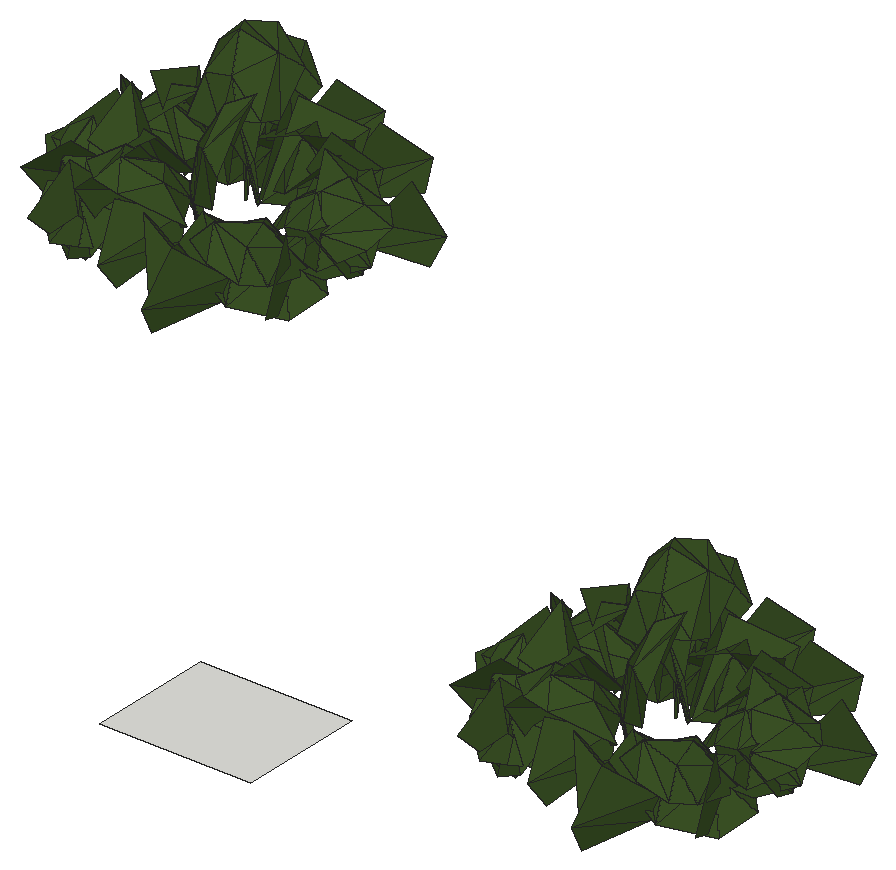
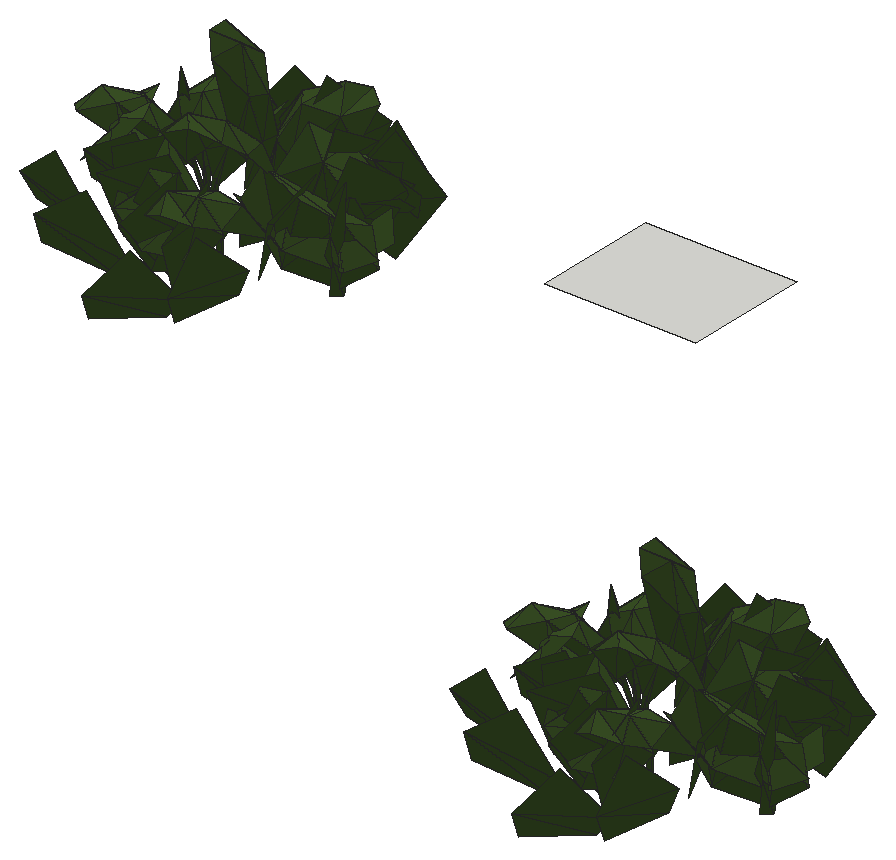
# SketchUp Ruby script. Lengths in inches.
U = 1.inch
M = Sketchup.active_model
def pt(a) = Geom::Point3d.new(a.map { |v| v * U })
def face(e, loops, mat)
  f = e.add_face(loops[0].map { |a| pt(a) })
  loops[1..].each { |l| e.add_face(l.map { |a| pt(a) }).erase! }
  f.material = f.back_material = mat if mat
  f
end
# faces: each face lists its corners as indices into pts; further lists are holes
def faces(e, pts, list, mat = nil) = list.each { |f| face(e, (f[0].is_a?(Array) ? f : [f]).map { |l| l.map { |i| pts[i] } }, mat) }
# xy, xz, yz: faces in a plane at the given z, y or x. An outline is a flat list of corners, or four numbers for a rectangle; further outlines are holes
def ring(l) = l.size == 4 ? [[l[0], l[1]], [l[2], l[1]], [l[2], l[3]], [l[0], l[3]]] : l.each_slice(2).to_a
def flat(e, list, mat, &to3) = list.each { |f| face(e, (f[0].is_a?(Array) ? f : [f]).map { |l| ring(l).map { |u, v| to3.(u, v) } }, mat) }
def xy(e, z, list, mat = nil) = flat(e, list, mat) { |x, y| [x, y, z] }
def xz(e, y, list, mat = nil) = flat(e, list, mat) { |x, z| [x, y, z] }
def yz(e, x, list, mat = nil) = flat(e, list, mat) { |y, z| [x, y, z] }
def lines(e, pts, list) = list.each { |a, b| e.add_line(pt(pts[a]), pt(pts[b])) }
# prism: a flat outline (further loops are holes) pulled along v
def prism(e, loops, v, mat = nil)
  f = face(e, loops, mat); d = Geom::Vector3d.new(v.map { |x| x * U })
  f.pushpull(f.normal.samedirection?(d) ? d.length : -d.length)
end
def box(e, o, s, mat = nil) = prism(e, [[o, [o[0] + s[0], o[1], o[2]], [o[0] + s[0], o[1] + s[1], o[2]], [o[0], o[1] + s[1], o[2]]]], [0, 0, s[2]], mat)
def at(x, y, z, deg = 0) = Geom::Transformation.translation(pt([x, y, z])) * Geom::Transformation.rotation(ORIGIN, Z_AXIS, deg.degrees)
def axes(o, x, y, z) = Geom::Transformation.new([*x, 0, *y, 0, *z, 0, *pt(o).to_a, 1])
def part(name) = M.definitions.add(name)
# library, detail: a bought-in or finely detailed component or shape, given as its bounding box
def library(name, o, s) = part(name).tap { |d| box(d.entities, o, s) }
def detail(e, o, s) = box(e.add_group.entities, o, s)
def put(e, d, t, mat = nil) = e.add_instance(d, t).tap { |i| i.material = mat if mat }
def group(e, t, mat = nil) = e.add_group.tap { |g| g.transformation = t; g.material = mat if mat }.entities
root = M.entities
M.materials.add("AM113_062_Tilia").color = [58, 81, 37]
xy(root,701.22,[[935.92,76.875,1160.625,265.5]])
p = [[1326.61,433.49,700.58],[1335.91,414.52,720.31],[1282.43,508.64,794.36],[1285.77,510.27,749.37],[165.99,1082.26,700.58],[175.28,1063.3,720.31],
  [121.81,1157.41,794.36],[125.14,1159.05,749.37],[1438.42,622.9,741.72],[1440.78,606.67,701.72],[1417.87,514.7,706.26],[277.79,1271.68,741.72],
  [280.15,1255.44,701.72],[257.25,1163.48,706.26],[1748.14,509.96,754.28],[1735.47,495.82,716.24],[1641.94,507.53,702.6875],[1627.76,518.58,727.05],
  [587.52,1158.74,754.28],[574.84,1144.59,716.24],[481.3125,1156.3,702.6875],[467.13,1167.35,727.05],[1678.41,298.07,824.98],[1678.04,260.96,728.32],
  [1664.82,334.88,702.98],[1591.24,362.94,765.53],[517.78,946.85,824.98],[517.41,909.74,728.32],[504.19,983.66,702.98],[430.62,1011.72,765.53],
  [1452.01,606.0625,704.71],[1436.57,598.83,730.18],[1504.92,698.75,754.5625],[1509.09,681.33,715.67],[291.38,1254.84,704.71],[275.95,1247.61,730.18],
  [344.29,1347.53,754.5625],[348.46,1330.1,715.67],[1405.95,373.7,766.25],[1329.15,333.13,705.79],[1288.375,289.91,783.48],[245.32,1022.47,766.25],
  [168.53,981.9,705.79],[127.75,938.6875,783.48],[1412.48,503.24,735.66],[251.85,1152.02,735.66],[1533.25,340.19,707.56],[1518.24,334.2,755.33],
  [1520.43,339.72,753.08],[1537.02,340.31,710.03],[1535.68,342.9,710.01],[1555.8,570.54,707.6],[1536.87,570.4,730.73],[1645.52,613.55,778.08],
  [1642.95,600.73,736.1],[372.625,988.97,707.56],[357.61,982.98,755.33],[359.81,988.49,753.08],[376.4,989.09,710.03],[375.06,991.67,710.01],
  [395.18,1219.3125,707.6],[376.25,1219.18,730.73],[484.89,1262.33,778.08],[482.33,1249.5,736.1],[1499.82,362.36,753.84],[1499.92,373,708.34],
  [1500.36,377.02,709.25],[339.2,1011.14,753.84],[339.29,1021.77,708.34],[339.74,1025.79,709.25],[1386.02,256.94,708.43],[1433.2,241.13,735.21],
  [1393.77,268.46,788.22],[1328.01,297.63,726.05],[1497.27,374.21,708.37],[1490.81,363.63,760.99],[1497.29,366.11,759.28],[225.4,905.72,708.43],
  [272.57,889.9,735.21],[233.14,917.24,788.22],[167.38,946.41,726.05],[336.64,1022.99,708.37],[330.18,1012.41,760.99],[336.67,1014.88,759.28],
  [1385.41,261.7,839.16],[1338.64,241.82,753.49],[1403.23,267.89,709.34],[1419.15,352.64,752.43],[224.78,910.47,839.16],[178.01,890.59,753.49],
  [242.61,916.67,709.34],[258.53,1001.42,752.43],[1523.14,331.27,760.7],[362.51,980.04,760.7],[1455.5,497.47,759.22],[1463.15,490.08,713.72],
  [1465.76,486.99,714.63],[1459.96,496.73,764.66],[1465.86,491.16,713.75],[1462.63,503.14,766.37],[294.875,1146.25,759.22],[302.52,1138.85,713.72],
  [305.13,1135.77,714.63],[299.33,1145.5,764.66],[305.23,1139.94,713.75],[302,1151.91,766.37],[1625.07,251.99,731.26],[1684.15,295.22,714.15],
  [1657.98,322.17,779.88],[1708.16,338.94,737.62],[464.4375,900.77,731.26],[523.52,944,714.15],[497.35,970.94,779.88],[547.53,987.71,737.62],
  [1583.43,375.32,752.05],[1566.11,390.15,714.72],[1563.87,392.87,717.45],[422.8,1024.09,752.05],[405.48,1038.93,714.72],[403.25,1041.64,717.45],
  [1563.51,388.96,715.42],[1578.09,368.2,759.62],[1580.38,374.86,758.97],[402.88,1037.74,715.42],[417.46,1016.97,759.62],[419.76,1023.64,758.97],
  [1500.56,255.27,811.84],[1561.13,292.5,716.8],[1485.75,346.05,716.44],[339.93,904.04,811.84],[400.51,941.27,716.8],[325.12,994.83,716.44],
  [1580.22,152.11,755.35],[1579.78,170.31,716.68],[1610.73,259.48,728.69],[419.6,800.89,755.35],[419.15,819.09,716.68],[450.1,908.25,728.69],
  [1536.8,219.18,726.5],[376.18,867.95,726.5],[1336.33,433.87,796.07],[1281.91,423.32,759.58],[1333.625,388.88,719.32],[1452.16,457.44,794.04],
  [175.71,1082.64,796.07],[121.28,1072.1,759.58],[173,1037.66,719.32],[291.53,1106.22,794.04],[1473.78,202.77,754.32],[1485.58,222.6875,720.33],
  [1514.89,308.5625,755.91],[1328.35,458.4375,815.82],[313.15,851.54,754.32],[324.95,871.46,720.33],[354.27,957.34,755.91],[167.72,1107.21,815.82],
  [1568.01,387.94,720.42],[1592.96,379.96,763.81],[1586.97,383.33,765.9],[1564.36,388.17,723.15],[407.39,1036.72,720.42],[432.33,1028.73,763.81],
  [426.34,1032.11,765.9],[403.73,1036.94,723.15],[1493.29,526.17,794.92],[1448.31,510.58,720.77],[1567.1,434.45,781.25],[1457.2,570.85,764],
  [332.66,1174.95,794.92],[287.68,1159.36,720.77],[406.48,1083.22,781.25],[296.58,1219.625,764],[1381.47,435.69,734.66],[1349.49,342.875,721.54],
  [1303.85,328.74,811.59],[220.85,1084.47,734.66],[188.87,991.65,721.54],[143.22,977.51,811.59],[1586.98,388.64,761.8],[1567.41,390.64,721.62],
  [426.35,1037.42,761.8],[406.79,1039.41,721.62],[1322.35,435.11,854.09],[1316.87,447.8,723.22],[1402.51,417.16,744.76],[1300.75,500.77,793.38],
  [161.73,1083.88,854.09],[156.24,1096.57,723.22],[241.88,1065.9375,744.76],[140.12,1149.54,793.38],[1490.9,537.0625,853.98],[1493.08,552.44,723.42],
  [1506.19,461.65,738.53],[1536.2,588.63,792.36],[330.28,1185.84,853.98],[332.45,1201.22,723.42],[345.56,1110.43,738.53],[375.57,1237.41,792.36],
  [1345.35,295.43,811.24],[1343.42,356.64,841.68],[1289.23,335.78,805.61],[184.72,944.2,811.24],[182.79,1005.41,841.68],[128.6,984.56,805.61],
  [1690.2,517.37,804.11],[529.57,1166.15,804.11],[1682.46,333.16,815.28],[1731.64,345.9375,764.14],[1698.99,415.79,727.27],[1701.08,396.03,811.58],
  [1666.04,441.33,825.18],[1662.48,474.11,755.35],[521.84,981.94,815.28],[571.02,994.71,764.14],[538.36,1064.57,727.27],[540.46,1044.81,811.58],
  [505.41,1090.1,825.18],[501.86,1122.89,755.35],[1524.64,444.25,750.71],[1586.08,519.4,727.68],[1596.8,556.02,825.08],[364.01,1093.03,750.71],
  [425.45,1168.18,727.68],[436.17,1204.79,825.08],[1332.16,437.6,728.36],[1285.84,390.25,765.55],[1338.74,330.03,789.98],[1347,396.1,806.91],
  [1398.75,382.46,832.35],[1465.52,394.21,792.07],[171.53,1086.38,728.36],[125.21,1039.03,765.55],[178.12,978.81,789.98],[186.37,1044.88,806.91],
  [238.12,1031.23,832.35],[304.89,1042.99,792.07],[1616.78,269.03,759],[456.15,917.8,759],[1472.2,651.3125,805.89],[311.57,1300.09,805.89],
  [1398.23,281.14,786.32],[1421.81,231.4,748.86],[1458.56,288.68,730.46],[1364.86,394.51,789.97],[1307.65,465.1,730.52],[1289.38,415.01,740.82],
  [1324.36,438.5,801.54],[1354.98,513.62,762.46],[237.61,929.92,786.32],[261.18,880.18,748.86],[297.93,937.46,730.46],[204.24,1043.29,789.97],
  [147.02,1113.88,730.52],[128.76,1063.78,740.82],[163.73,1087.28,801.54],[194.35,1162.4,762.46],[1504.57,568.33,730.73],[1452.31,561.0625,745.02],
  [1492.2,538.72,801.25],[1570.86,547.59,755.99],[1588.45,586.91,817.61],[343.94,1217.1,730.73],[291.68,1209.84,745.02],[331.57,1187.5,801.25],
  [410.23,1196.37,755.99],[427.83,1235.6875,817.61],[1541.05,314.99,800.37],[1560.82,245.55,797.22],[1612.51,291.64,800.44],[380.43,963.77,800.37],
  [400.1875,894.33,797.22],[451.88,940.42,800.44],[1473.06,366.21,781.8],[1429.77,286.17,732.5],[1410.46,238.71,819.34],[312.43,1014.99,781.8],
  [269.15,934.95,732.5],[249.83,887.49,819.34],[1371.32,241.83,732.55],[1317.31,291.12,750.31],[210.69,890.61,732.55],[156.68,939.9,750.31],
  [1347.9,395.03,862.42],[187.28,1043.8,862.42],[1453.46,275.71,782.99],[292.83,924.49,782.99],[1439.04,568.99,799.38],[278.41,1217.77,799.38],
  [1425.71,425.16,759.48],[1388.48,514.92,737.1875],[1355.6,538.56,833],[265.08,1073.9375,759.48],[227.85,1163.7,737.1875],[194.97,1187.33,833],
  [1564.44,475.96,737.43],[1544.77,478.44,759.28],[1656.14,507.1875,813.76],[1653.57,494.59,771.66],[403.8125,1124.74,737.43],[384.14,1127.22,759.28],
  [495.51,1155.96,813.76],[492.94,1143.37,771.66],[1660.44,389.51,738.49],[499.82,1038.28,738.49],[1476.72,514.23,787.18],[1448.46,600.73,737.88],
  [1427.33,647.41,824.72],[316.09,1163.01,787.18],[287.83,1249.5,737.88],[266.7,1296.18,824.72],[1325.27,382.41,773.14],[164.65,1031.1875,773.14],
  [1632.35,347.61,744.61],[1628.35,353.95,781.24],[1667.46,315.29,796.85],[1677.61,348.86,752.36],[471.72,996.39,744.61],[467.73,1002.72,781.24],
  [506.83,964.0625,796.85],[516.98,997.64,752.36],[1441.45,513.08,775.49],[280.82,1161.86,775.49],[1377.06,386.95,886],[1432.41,342.61,790.73],
  [1404.05,423.31,745.4],[216.43,1035.72,886],[271.78,991.38,790.73],[243.42,1072.08,745.4],[1505.52,442.3,790.5],[1516.93,445.81,745.54],
  [1519.89,442.97,745.76],[344.89,1091.07,790.5],[356.31,1094.58,745.54],[359.27,1091.74,745.76],[1637.79,323.52,766.8],[1709.72,329.4,762.91],
  [1715.7,410.44,745.63],[1676.57,380.4,805.74],[1656.39,432.39,821.15],[1686.32,474.98,774.7],[477.16,972.29,766.8],[549.1,978.17,762.91],
  [555.08,1059.22,745.63],[515.94,1029.17,805.74],[495.76,1081.16,821.15],[525.7,1123.75,774.7],[1509.69,440.95,796.125],[1519.44,447.15,746.33],
  [349.07,1089.73,796.125],[358.82,1095.93,746.33],[1511.3,447.02,800.32],[350.68,1095.79,800.32],[1360.15,320.6,806.56],[1302.88,359.62,806.28],
  [199.52,969.37,806.56],[142.26,1008.4,806.28],[1520.73,518.52,859.1],[360.1,1167.29,859.1],[1604.1875,352.33,798.3125],[443.5625,1001.1,798.3125],
  [1678.22,263.48,771.29],[517.59,912.25,771.29],[1504.83,334.66,810.43],[1504.15,362.125,813.85],[344.21,983.4375,810.43],[343.52,1010.9,813.85],
  [1495.83,346.74,811.32],[1513.65,326.46,803.92],[335.2,995.52,811.32],[353.02,975.24,803.92],[1512.04,316.23,787.85],[1461.31,250.43,818.53],
  [351.41,965,787.85],[300.68,899.21,818.53],[1583.74,203.1,817.12],[423.11,851.875,817.12],[1633.27,493.68,808.08],[472.64,1142.45,808.08],
  [1543.79,526,831.95],[1565.53,465.11,846.5],[1611.08,509.75,834.6],[383.16,1174.77,831.95],[404.91,1113.88,846.5],[450.46,1158.53,834.6],
  [1640.36,359.82,757.68],[1693.88,335.37,765.71],[1690.43,349.4,808.05],[1622.41,365.7,786.55],[479.73,1008.59,757.68],[533.25,984.14,765.71],
  [529.8,998.18,808.05],[461.78,1014.48,786.55],[1446.92,511.12,816.7],[1419.94,512.15,809.3],[286.29,1159.9,816.7],[259.32,1160.93,809.3],
  [1594.58,488.49,849.45],[433.95,1137.27,849.45],[1352.16,452.87,862.78],[191.53,1101.64,862.78],[1580.81,339.61,790.05],[1295.96,474.5,761.3],
  [420.18,988.39,790.05],[135.33,1123.27,761.3],[1525.62,317.35,805.03],[364.99,966.12,805.03],[1470.87,352.28,798.7],[310.24,1001.05,798.7],
  [1351.43,518.61,790.52],[190.8,1167.39,790.52],[1615.55,384.76,810.3125],[1618.84,412.16,810.4],[454.93,1033.53,810.3125],[458.21,1060.93,810.4],
  [1509.1,581.92,762.04],[1575.07,552.04,784.05],[348.47,1230.69,762.04],[414.44,1200.8125,784.05],[1357.57,477.53,837.21],[1420.69,468.34,857.14],
  [1402.62,529.64,846.43],[196.94,1126.3,837.21],[260.07,1117.12,857.14],[241.99,1178.42,846.43],[1739,373.92,791.96],[578.37,1022.69,791.96],
  [1363.62,289.24,844.33],[202.99,938.01,844.33],[1468.12,525.42,804.08],[307.49,1174.19,804.08],[1590.01,462.04,799.33],[429.39,1110.82,799.33],
  [1569.3,317.82,769.61],[1563.37,262.34,795.01],[1590,272.97,822.8125],[408.68,966.6,769.61],[402.74,911.12,795.01],[429.37,921.75,822.8125],
  [1658.42,234.71,780.29],[1647.9,262.39,813.4],[497.79,883.48,780.29],[487.27,911.17,813.4],[1511.0625,279.72,844.28],[1543.64,281.48,796.79],
  [1512.42,309.35,773.17],[350.43,928.5,844.28],[383.02,930.26,796.79],[351.79,958.125,773.17],[1649.93,494.24,817.93],[489.31,1143.01,817.93],
  [1408.375,524.83,778.55],[1387.82,546.21,849.66],[1366.67,521.36,802.17],[247.75,1173.6,778.55],[227.2,1194.98,849.66],[206.05,1170.13,802.17],
  [1624.69,428.37,779.73],[1665.77,432.83,840.375],[1633.9,464.29,814.14],[464.0625,1077.15,779.73],[505.14,1081.61,840.375],[473.27,1113.07,814.14],
  [1615.98,228.17,795.98],[455.35,876.94,795.98],[1629.79,317.17,816.89],[1540.68,499.26,816.62],[1607.85,483.49,825.05],[469.17,965.95,816.89],
  [380.06,1148.04,816.62],[447.22,1132.27,825.05],[1472.43,282.76,878.55],[1447.45,340.52,781.82],[1401.91,316.58,819.52],[1427.11,313.05,852.14],
  [311.81,931.54,878.55],[286.82,989.29,781.82],[241.29,965.36,819.52],[266.48,961.82,852.14],[1656.14,393.39,835.36],[495.52,1042.17,835.36],
  [1416.62,572.13,883.93],[1469.79,584.16,857.52],[1475.71,550.5,787.2],[1489.69,600.01,824.91],[255.99,1220.91,883.93],[309.16,1232.9375,857.52],
  [315.08,1199.27,787.2],[329.07,1248.78,824.91],[1406.38,319.72,827.68],[245.75,968.5,827.68],[1380.6875,462.88,823.25],[1491.56,442.11,848.91],
  [1465.26,441.53,838.16],[1424.9375,514.94,838.2],[220.06,1111.66,823.25],[330.93,1090.89,848.91],[304.63,1090.3,838.16],[264.3125,1163.72,838.2],
  [1371.91,311.77,839.23],[211.29,960.54,839.23],[1741.64,417.26,805.26],[581.02,1066.03,805.26],[1447.21,347.06,853.62],[286.58,995.83,853.62],
  [1480.54,232.3,839.69],[319.91,881.08,839.69],[1486.69,312.26,848.41],[326.06,961.04,848.41],[1511.2,460.91,844.78],[350.57,1109.68,844.78],
  [1374.4375,600.99,845.07],[213.81,1249.76,845.07],[1525.77,380.27,803.38],[1508.35,383.51,880.83],[1505.3125,414.64,831.85],[365.14,1029.04,803.38],
  [347.73,1032.29,880.83],[344.69,1063.41,831.85],[1428.2,541.49,853.79],[267.58,1190.26,853.79],[1549.99,303.47,890.44],[1509.85,344,867.93],
  [1554.57,314.01,808.77],[389.36,952.24,890.44],[349.23,992.77,867.93],[393.95,962.78,808.77],[1713.42,400.5625,832.9375],[1717.78,442.63,814.85],
  [552.8,1049.34,832.9375],[557.16,1091.41,814.85],[1610,455.01,847.66],[449.375,1103.79,847.66],[1580.53,291.99,871.21],[419.9,940.77,871.21],
  [1453.93,458.8125,811.24],[1426.2,461.71,883.54],[1411.82,445.625,826.51],[293.3,1107.59,811.24],[265.58,1110.49,883.54],[251.2,1094.4,826.51],
  [1412.04,259.33,849.95],[251.41,908.11,849.95],[1441.2,632.07,855.33],[280.57,1280.84,855.33],[1405.4375,513.42,895.61],[244.81,1162.2,895.61],
  [1552.22,397.38,923.14],[391.6,1046.16,923.14],[1466.46,461.03,891.91],[1501.14,505.82,916.05],[1516.14,489.32,838.1875],[1520.52,530.19,893.09],
  [305.83,1109.81,891.91],[340.51,1154.59,916.05],[355.51,1138.1,838.1875],[359.89,1178.97,893.09],[1445.76,230.11,849.17],[1458.45,264.2,867.94],
  [285.13,878.88,849.17],[297.83,912.98,867.94],[1412.78,595.05,873.33],[1396.79,627.73,854.55],[252.16,1243.82,873.33],[236.16,1276.5,854.55],
  [1541.84,354.25,928.54],[381.21,1003.03,928.54],[1584.58,331.3,934.07],[423.96,980.07,934.07],[1442.37,506.21,926.39],[281.74,1154.99,926.39],
  [1573.6,373.88,943.9],[412.97,1022.65,943.9],[1466.21,548.6875,925.84],[305.59,1197.46,925.84],[1423.07,539.54,917.03],[262.44,1188.3125,917.03]]
faces(root,p,[[0,1,2],[2,3,0],[4,5,6],[6,7,4],[8,9,10],[11,12,13],[14,15,16],[16,17,14],
  [18,19,20],[20,21,18],[22,23,24],[22,24,25],[26,27,28],[26,28,29],[30,31,32],[32,33,30],
  [34,35,36],[36,37,34],[38,39,40],[41,42,43],[10,44,8],[13,45,11],[46,47,48],[47,46,49],
  [48,50,46],[51,52,53],[53,54,51],[55,56,57],[56,55,58],[57,59,55],[60,61,62],[62,63,60],
  [64,65,66],[67,68,69],[70,71,72],[73,70,72],[74,75,76],[76,66,74],[77,78,79],[80,77,79],
  [81,82,83],[83,69,81],[84,85,86],[84,86,87],[66,76,64],[88,89,90],[88,90,91],[69,83,67],
  [49,92,47],[58,93,56],[94,95,96],[97,96,98],[98,99,97],[100,101,102],[103,102,104],[104,105,103],
  [106,107,108],[107,109,108],[110,111,112],[111,113,112],[96,97,94],[102,103,100],[114,115,116],[117,118,119],
  [120,121,122],[122,116,120],[123,124,125],[125,119,123],[126,127,128],[129,130,131],[132,133,134],[135,136,137],
  [126,138,127],[129,139,130],[116,122,114],[119,125,117],[140,141,142],[140,142,143],[144,145,146],[144,146,147],
  [148,149,150],[1,151,2],[152,153,154],[5,155,6],[156,157,158],[158,159,156],[160,161,162],[162,163,160],
  [164,165,166],[164,167,165],[168,169,170],[168,171,169],[172,173,174],[175,176,177],[178,179,159],[180,181,163],
  [159,158,178],[182,183,184],[182,185,183],[163,162,180],[186,187,188],[186,189,187],[190,191,192],[190,193,191],
  [194,195,196],[194,197,195],[72,198,73],[73,198,199],[199,200,73],[79,201,80],[80,201,202],[202,203,80],
  [17,204,14],[21,205,18],[206,207,208],[208,209,206],[210,209,208],[208,211,210],[212,213,214],[214,215,212],
  [216,215,214],[214,217,216],[218,219,220],[221,222,223],[224,225,226],[226,227,224],[228,229,224],[224,227,228],
  [230,231,232],[232,233,230],[234,235,230],[230,233,234],[134,236,132],[137,237,135],[31,238,32],[35,239,36],
  [240,241,242],[240,242,243],[244,245,246],[247,244,246],[248,249,250],[248,250,251],[252,253,254],[255,252,254],
  [256,257,258],[259,256,258],[52,260,53],[261,262,263],[264,261,263],[61,265,62],[266,267,106],[106,268,266],
  [108,268,106],[269,270,110],[110,271,269],[112,271,110],[272,273,274],[275,276,277],[278,241,240],[279,278,240],
  [280,249,248],[281,280,248],[282,172,174],[283,175,177],[72,71,284],[79,78,285],[44,286,8],[45,287,11],
  [288,289,290],[291,292,293],[294,295,296],[296,297,294],[298,299,300],[300,301,298],[108,109,302],[112,113,303],
  [304,305,306],[307,308,309],[108,302,266],[112,303,269],[246,245,310],[254,253,311],[312,313,314],[314,315,312],
  [316,317,318],[318,319,316],[258,257,320],[263,262,321],[322,323,324],[325,326,327],[328,329,330],[331,332,333],
  [334,335,336],[336,337,334],[338,337,336],[336,339,338],[340,341,342],[342,343,340],[344,343,342],[342,345,344],
  [330,346,328],[346,330,347],[333,348,331],[348,333,349],[347,350,346],[349,351,348],[240,352,279],[243,353,279],
  [279,352,243],[248,354,281],[251,355,281],[281,354,251],[356,218,220],[357,221,223],[114,122,358],[358,313,114],
  [117,125,359],[359,317,117],[360,315,314],[361,319,318],[48,47,362],[362,363,48],[57,56,364],[364,365,57],
  [366,367,64],[64,76,366],[368,369,67],[67,83,368],[370,371,148],[150,370,148],[372,373,152],[154,372,152],
  [236,374,132],[362,47,92],[237,375,135],[364,56,93],[211,376,210],[217,377,216],[259,378,379],[379,380,259],
  [258,378,259],[264,381,382],[382,383,264],[263,381,264],[384,385,386],[386,387,384],[388,389,390],[390,391,388],
  [358,122,121],[359,125,124],[94,97,392],[392,393,94],[100,103,394],[394,395,100],[366,76,75],[295,396,296],
  [368,83,82],[299,397,300],[398,288,290],[399,291,293],[121,400,358],[401,141,140],[124,402,359],[403,145,144],
  [92,404,362],[93,405,364],[75,406,366],[82,407,368],[408,401,140],[409,403,144],[178,158,410],[410,411,178],
  [180,162,412],[412,413,180],[414,167,164],[415,414,164],[416,171,168],[417,416,168],[246,418,247],[419,420,247],
  [247,418,419],[254,421,255],[422,423,255],[255,421,422],[157,387,410],[410,158,157],[161,391,412],[412,162,161],
  [392,97,99],[394,103,105],[386,385,424],[390,389,425],[426,38,40],[427,41,43],[99,428,392],[105,429,394],
  [338,430,334],[334,337,338],[344,431,340],[340,343,344],[432,433,434],[434,400,432],[435,436,437],[437,402,435],
  [438,360,439],[439,360,314],[440,361,441],[441,361,318],[246,310,419],[254,311,422],[442,443,444],[444,367,442],
  [445,446,447],[447,369,445],[339,448,338],[345,449,344],[258,320,379],[263,321,382],[450,393,451],[451,452,450],
  [453,395,454],[454,455,453],[456,411,457],[457,458,456],[459,413,460],[460,461,459],[266,268,108],[269,271,112],
  [434,462,438],[438,439,434],[437,463,440],[440,441,437],[464,314,313],[464,313,358],[166,465,164],[415,465,166],
  [166,466,415],[467,318,317],[467,317,359],[170,468,168],[417,468,170],[170,469,417],[470,272,274],[471,472,473],
  [473,406,471],[474,275,277],[475,476,477],[477,407,475],[72,284,199],[79,285,202],[164,465,415],[168,468,417],
  [243,352,240],[251,354,248],[387,386,478],[478,410,387],[391,390,479],[479,412,391],[480,304,306],[481,428,482],
  [482,483,481],[484,307,309],[485,429,486],[486,487,485],[199,198,72],[202,201,79],[400,434,464],[464,358,400],
  [226,488,228],[228,227,226],[402,437,467],[467,359,402],[232,489,234],[234,233,232],[140,490,408],[328,346,491],
  [491,492,328],[143,493,408],[408,490,143],[144,494,409],[331,348,495],[495,496,331],[147,497,409],[409,494,147],
  [322,498,323],[325,499,326],[386,424,500],[390,425,501],[228,502,229],[234,503,235],[143,490,140],[147,494,144],
  [434,433,462],[437,436,463],[491,346,350],[495,348,351],[504,443,442],[505,446,445],[464,439,314],[467,441,318],
  [406,473,506],[506,366,406],[407,477,507],[507,368,407],[338,448,430],[344,449,431],[350,508,491],[351,509,495],
  [379,378,258],[382,381,263],[419,418,246],[422,421,254],[510,452,451],[511,455,454],[512,363,513],[513,514,512],
  [515,365,516],[516,517,515],[506,442,367],[506,367,366],[507,445,369],[507,369,368],[518,392,428],[428,481,518],
  [519,394,429],[429,485,519],[404,520,521],[520,404,522],[521,362,404],[405,523,524],[523,405,525],[524,364,405],
  [500,526,386],[500,527,526],[501,528,390],[501,529,528],[386,526,478],[210,376,530],[390,528,479],[216,377,531],
  [522,532,520],[525,533,523],[518,393,392],[518,451,393],[519,395,394],[519,454,395],[478,411,410],[479,413,412],
  [521,363,362],[478,457,411],[524,365,364],[479,460,413],[534,492,535],[535,536,534],[537,496,538],[538,539,537],
  [206,209,210],[212,215,216],[434,439,464],[437,441,467],[521,513,363],[524,516,365],[527,458,457],[529,461,460],
  [526,527,457],[528,529,460],[210,530,206],[216,531,212],[473,472,540],[477,476,541],[481,483,542],[485,487,543],
  [544,536,535],[545,539,538],[488,502,228],[489,503,234],[546,514,513],[547,517,516],[478,526,457],[479,528,460],
  [548,535,492],[548,492,491],[549,508,550],[550,551,549],[552,538,496],[552,496,495],[553,509,554],[554,555,553],
  [556,504,557],[557,504,442],[558,505,559],[559,505,445],[506,557,442],[507,559,445],[548,491,508],[508,549,548],
  [552,495,509],[509,553,552],[560,510,451],[561,510,560],[562,511,454],[563,511,562],[473,557,506],[477,559,507],
  [473,540,556],[556,557,473],[477,541,558],[558,559,477],[518,560,451],[519,562,454],[481,560,518],[485,562,519],
  [481,542,561],[561,560,481],[485,543,563],[563,562,485],[520,564,521],[521,564,513],[523,565,524],[524,565,516],
  [520,532,566],[523,533,567],[564,546,513],[565,547,516],[548,568,535],[568,544,535],[552,569,538],[569,545,538],
  [570,564,520],[520,566,570],[571,565,523],[523,567,571],[549,568,548],[553,569,552],[549,551,572],[553,555,573],
  [574,544,568],[575,545,569],[549,572,574],[574,568,549],[553,573,575],[575,569,553],[570,546,564],[571,547,565]],"AM113_062_Tilia")
